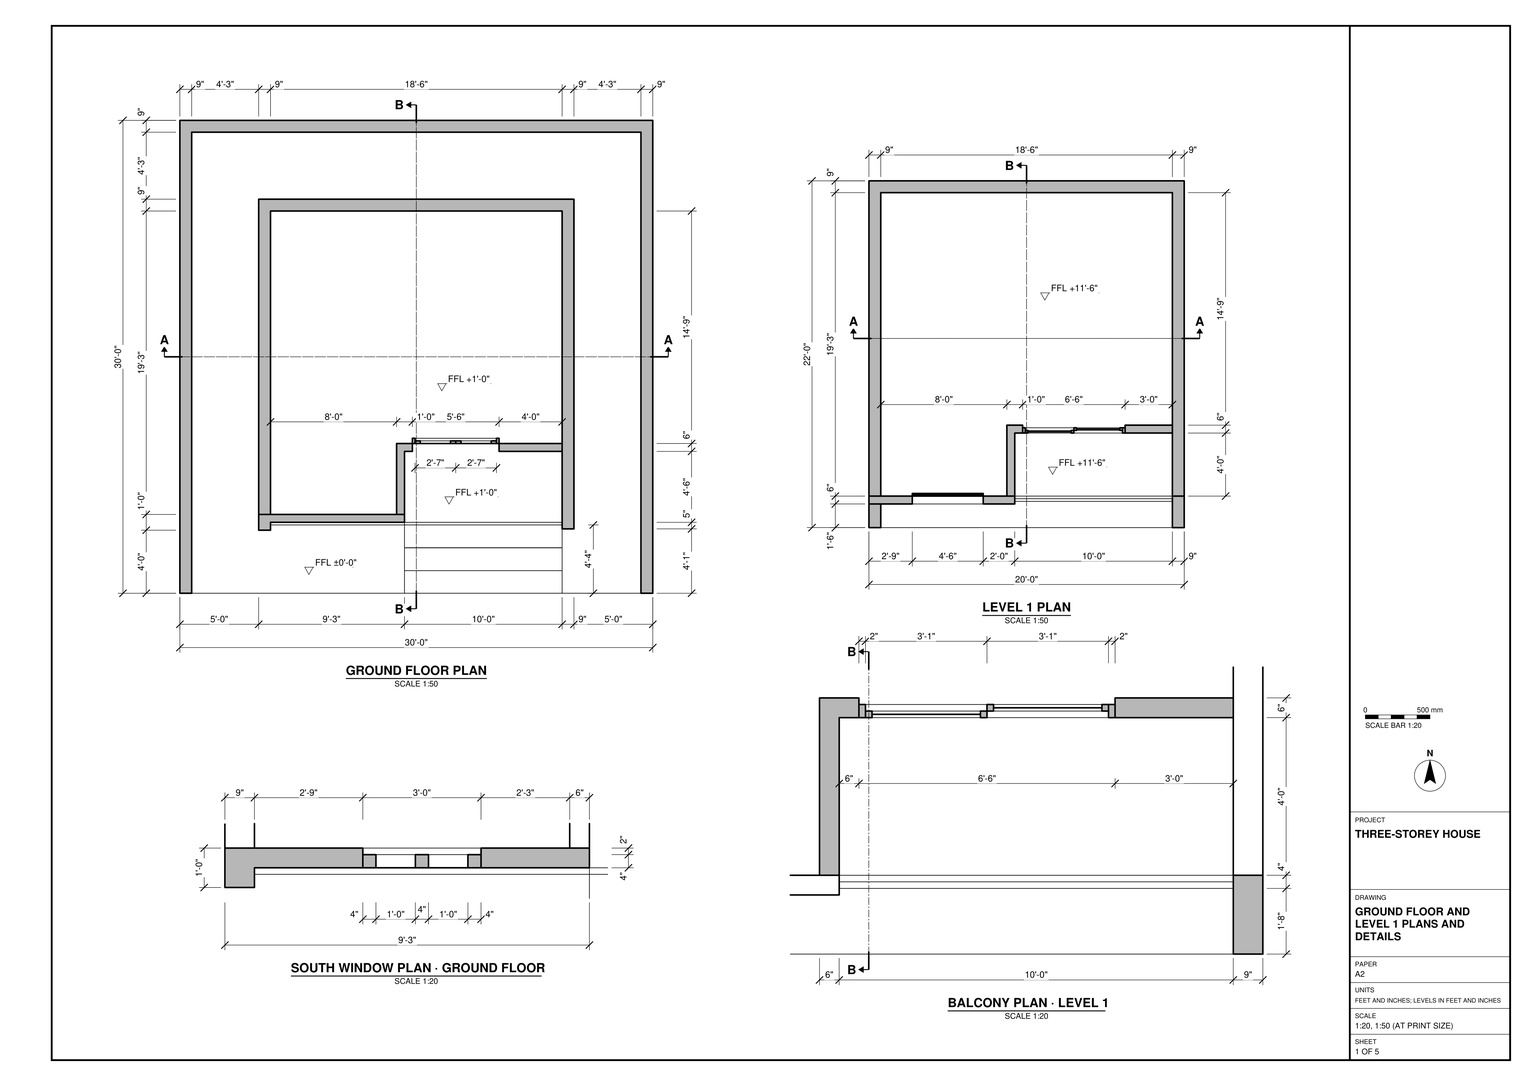
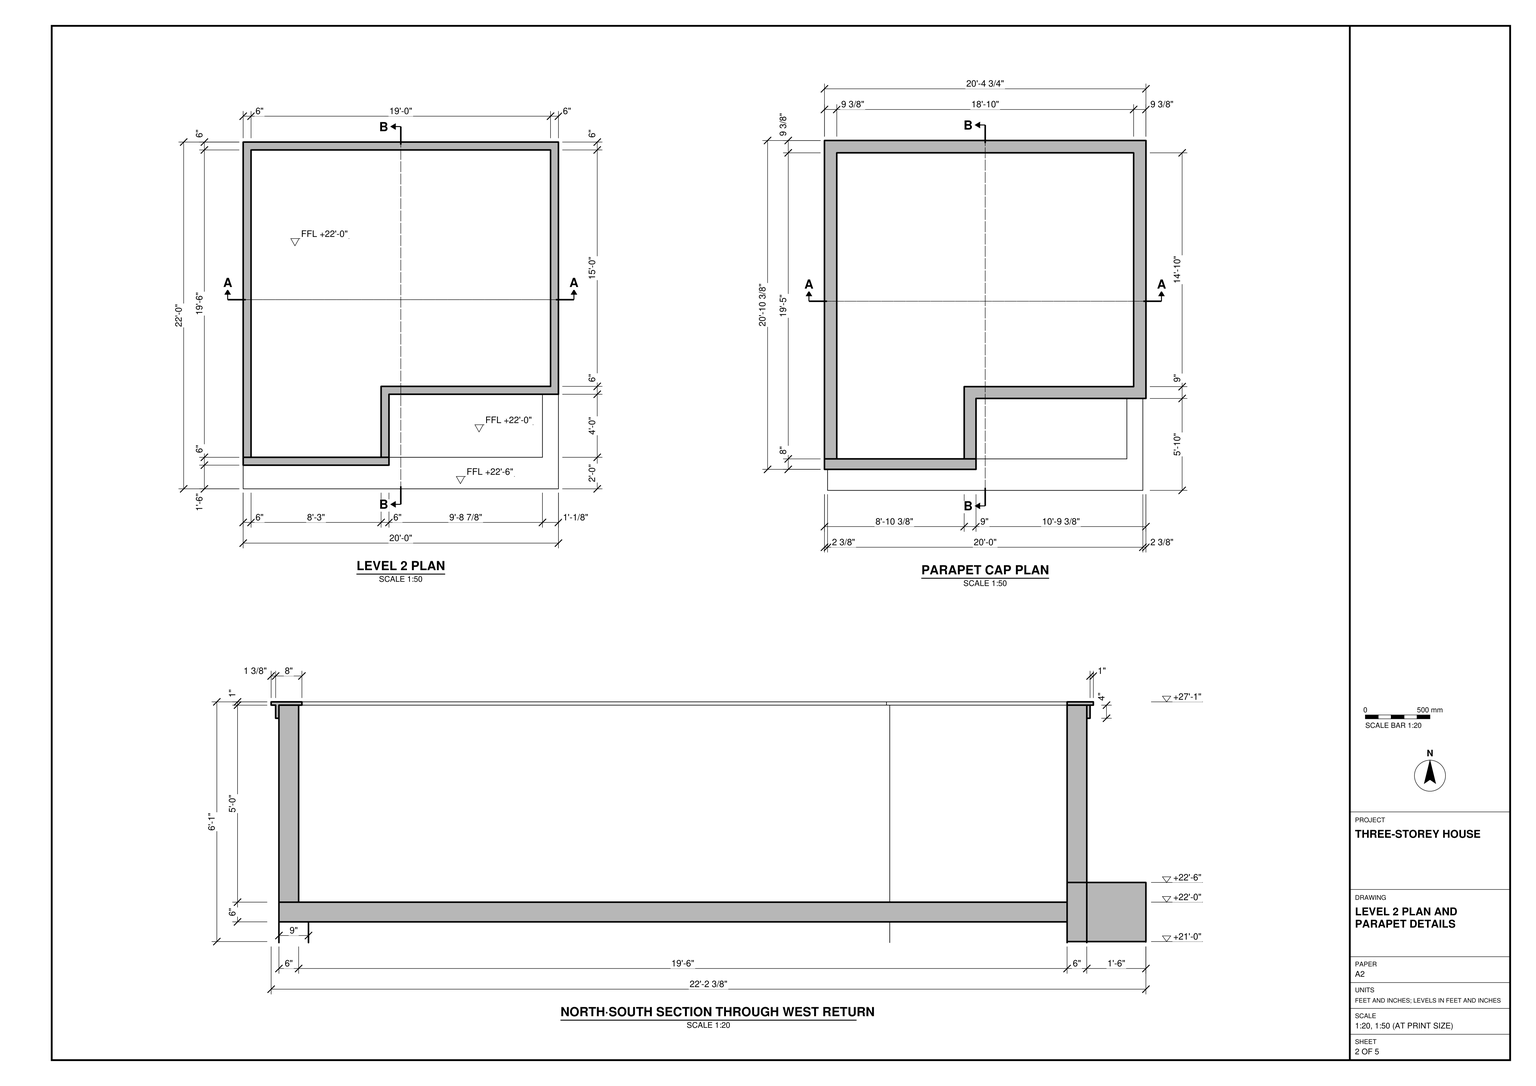
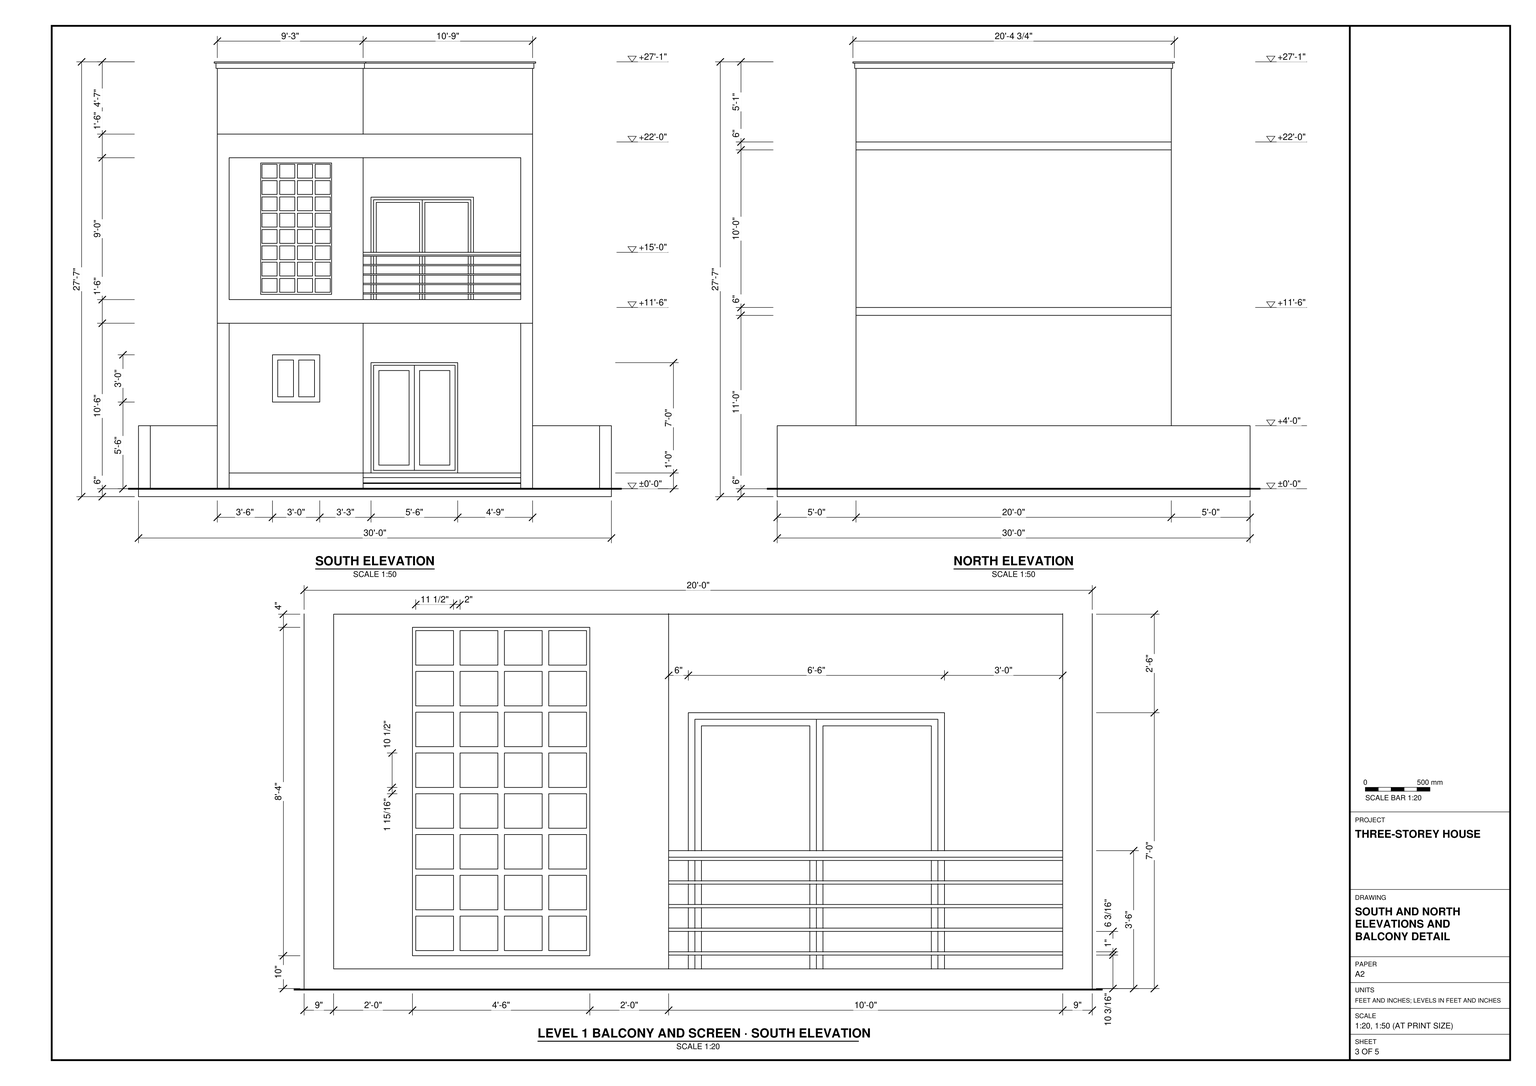
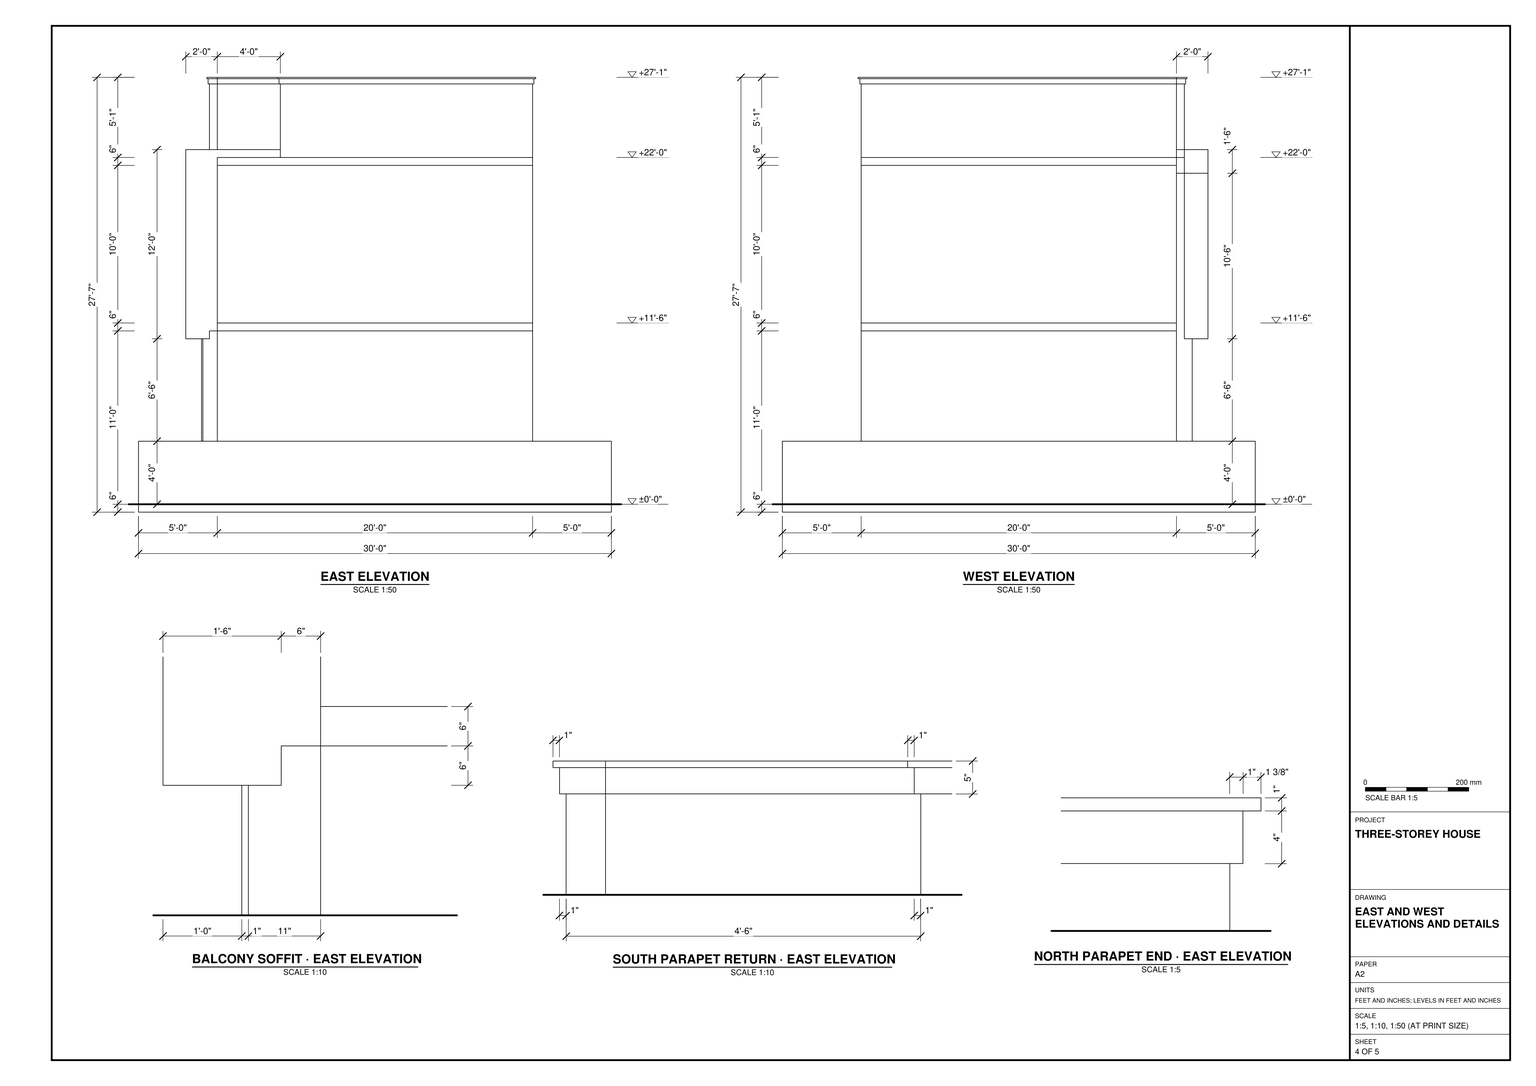
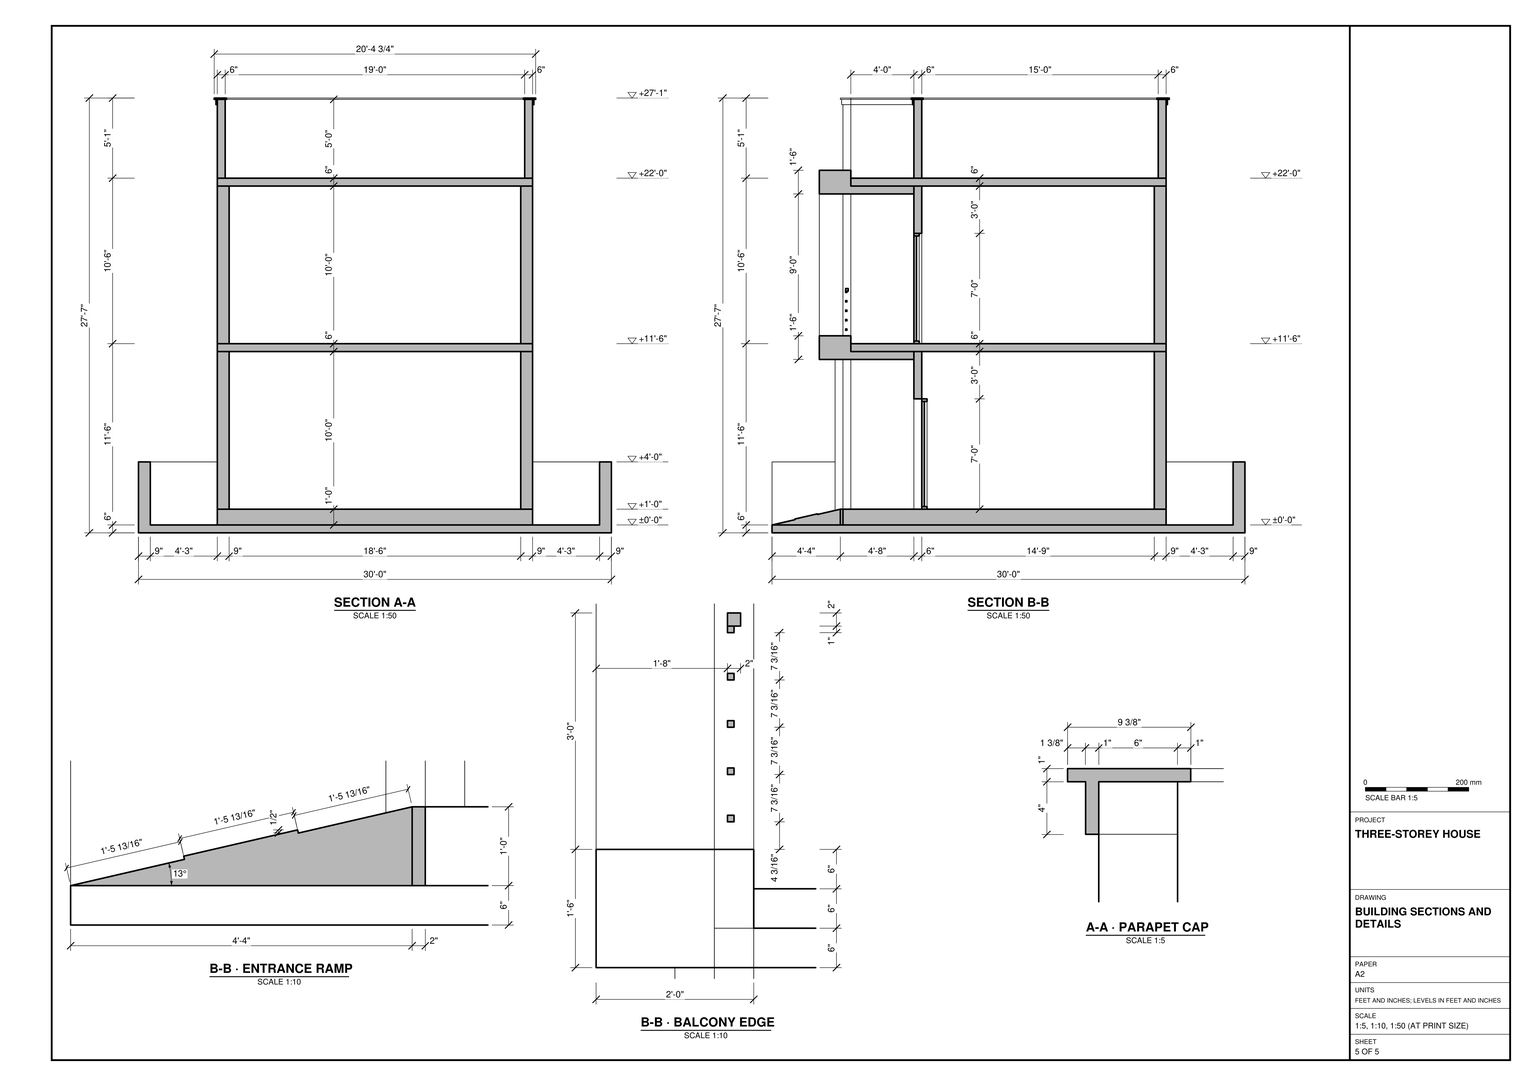
Build the house and its walled site in SketchUp from task_files/diagram_01.pdf. Work in feet and inches. The model is 30'-0" wide, 30'-0" deep and 27'-7" high, measured from the underside of the base slab to the top of the parapet cap. Use ±0'-0" as the ground datum, with Level 1 at +11'-6" and Level 2 at +22'-0". The finished ground floor is raised to +1'-0" above the approach.

Place the house between the low site walls, leaving the approach open to the south. Model the entrance steps, floor slabs and wall returns, following the wall thicknesses in plan. On the south face, place the small divided window to the left of the recessed entrance. Above it, build the tall grid screen beside the balcony, with the two-panel balcony doorway set back behind the horizontal railing. At roof level, follow the stepped parapet outline and carry the projecting cap around its returns.

Keep shell elements such as walls, slabs and roof, and each furniture or joinery piece shown, in separate groups or components. Use components for repeated parts. Any decor or loose items shown may be suitable library components. Save one SketchUp model as output_files/three_storey_house_with_a_recessed_south_balcony.skp.

# SketchUp Ruby script. Lengths in inches.
U = 1.inch
M = Sketchup.active_model
def pt(a) = Geom::Point3d.new(a.map { |v| v * U })
def face(e, loops, mat)
  f = e.add_face(loops[0].map { |a| pt(a) })
  loops[1..].each { |l| e.add_face(l.map { |a| pt(a) }).erase! }
  f.material = f.back_material = mat if mat
  f
end
# faces: each face lists its corners as indices into pts; further lists are holes
def faces(e, pts, list, mat = nil) = list.each { |f| face(e, (f[0].is_a?(Array) ? f : [f]).map { |l| l.map { |i| pts[i] } }, mat) }
# xy, xz, yz: faces in a plane at the given z, y or x. An outline is a flat list of corners, or four numbers for a rectangle; further outlines are holes
def ring(l) = l.size == 4 ? [[l[0], l[1]], [l[2], l[1]], [l[2], l[3]], [l[0], l[3]]] : l.each_slice(2).to_a
def flat(e, list, mat, &to3) = list.each { |f| face(e, (f[0].is_a?(Array) ? f : [f]).map { |l| ring(l).map { |u, v| to3.(u, v) } }, mat) }
def xy(e, z, list, mat = nil) = flat(e, list, mat) { |x, y| [x, y, z] }
def xz(e, y, list, mat = nil) = flat(e, list, mat) { |x, z| [x, y, z] }
def yz(e, x, list, mat = nil) = flat(e, list, mat) { |y, z| [x, y, z] }
def lines(e, pts, list) = list.each { |a, b| e.add_line(pt(pts[a]), pt(pts[b])) }
# prism: a flat outline (further loops are holes) pulled along v
def prism(e, loops, v, mat = nil)
  f = face(e, loops, mat); d = Geom::Vector3d.new(v.map { |x| x * U })
  f.pushpull(f.normal.samedirection?(d) ? d.length : -d.length)
end
def box(e, o, s, mat = nil) = prism(e, [[o, [o[0] + s[0], o[1], o[2]], [o[0] + s[0], o[1] + s[1], o[2]], [o[0], o[1] + s[1], o[2]]]], [0, 0, s[2]], mat)
def at(x, y, z, deg = 0) = Geom::Transformation.translation(pt([x, y, z])) * Geom::Transformation.rotation(ORIGIN, Z_AXIS, deg.degrees)
def axes(o, x, y, z) = Geom::Transformation.new([*x, 0, *y, 0, *z, 0, *pt(o).to_a, 1])
def part(name) = M.definitions.add(name)
# library, detail: a bought-in or finely detailed component or shape, given as its bounding box
def library(name, o, s) = part(name).tap { |d| box(d.entities, o, s) }
def detail(e, o, s) = box(e.add_group.entities, o, s)
def put(e, d, t, mat = nil) = e.add_instance(d, t).tap { |i| i.material = mat if mat }
def group(e, t, mat = nil) = e.add_group.tap { |g| g.transformation = t; g.material = mat if mat }.entities
root = M.entities
M.materials.add("[Black Lines 2]").color = [239, 239, 239]
M.materials.add("[Carpet Berber Pattern Gray]").color = [165, 165, 165]
M.materials.add("[Carpet Diamond Yellow]").color = [226, 217, 124]
M.materials.add("[Color M05]").color = [114, 114, 114]
M.materials.add("[Metal Seamed]").color = [118, 119, 115]
M.materials.add("[Roofing Slate Tan]1").color = [200, 175, 128]
M.materials.add("[Tile Travertine 2 inch]").color = [181, 178, 172]
M.materials.add("[Translucent Glass Blue]").color = [100, 149, 237]
M.materials["[Translucent Glass Blue]"].alpha = 0.5
M.materials.add("[Windmill]").color = [236, 236, 236]
M.materials.add("[Wood Floor]").color = [155, 105, 61]
c1 = library("Group\#10",[0,0,0],[54,2,100])
c2 = part("Group\#19")
xz(c2.entities,1,[[2,2,35,78]],"[Translucent Glass Blue]")
g1 = group(c2.entities,at(0,0,0))
prism(g1,[[[0,0,0],[37,0,0],[37,0,80],[0,0,80]],[[2,0,78],[35,0,78],[35,0,2],[2,0,2]]],[0,2,0])
prism(root,[[[171,0,6],[171,17.33,10],[171,17.22,10.49],[171,34.55,14.49],[171,34.67,14],[171,52,18],[171,52,6]]],[120,0,0],"[Tile Travertine 2 inch]")
p = [[171,54,18],[171,52,18]]
lines(root,p,[[0,1]])
g2 = group(root,at(0,0,0),"[Carpet Diamond Yellow]")
xy(g2,0,[[0,0,360,360]],"[Carpet Berber Pattern Gray]")
xy(g2,6,[[9,0,351,351]],"[Windmill]")
xy(g2,54,[[0,0,9,0,9,351,351,351,351,0,360,0,360,360,0,360]],"[Carpet Berber Pattern Gray]")
xz(g2,0,[[0,0,360,0,360,54,351,54,351,6,9,6,9,54,0,54]],"[Carpet Berber Pattern Gray]")
xz(g2,351,[[9,6,351,54]],"[Carpet Berber Pattern Gray]")
xz(g2,360,[[0,0,360,54]],"[Carpet Berber Pattern Gray]")
yz(g2,0,[[0,0,360,54]],"[Carpet Berber Pattern Gray]")
yz(g2,9,[[0,6,351,54]],"[Carpet Berber Pattern Gray]")
yz(g2,351,[[0,6,351,54]],"[Carpet Berber Pattern Gray]")
yz(g2,360,[[0,0,360,54]],"[Carpet Berber Pattern Gray]")
g3 = group(root,at(60,60,6),"[Color M05]")
xy(g3,0,[[0,-8,240,-6],[0,-6,240,240]])
xy(g3,12,[[0,-8,240,-6],[0,-6,240,240]])
xz(g3,-8,[[0,0,240,12]])
xz(g3,-6,[[0,0,240,12]])
xz(g3,240,[[0,0,240,12]])
yz(g3,0,[[-8,0,-6,12],[-6,0,240,12]])
yz(g3,240,[[-8,0,-6,12],[-6,0,240,12]])
g4 = group(root,at(60,60,18),"[Color M05]")
xy(g4,-12,[[231,-11,240,-8]])
xy(g4,0,[[231,-8,231,231,9,231,9,0,0,0,0,240,240,240,240,-8],[105,0,105,54,117,54,117,48,111,48,111,0],[183,48,231,54]])
xy(g4,84,[[117,48,183,54]])
xy(g4,114,[[231,-11,240,-6]])
xy(g4,120,[[231,-6,240,-6,240,240,0,240,0,0,9,0,9,231,231,231],[105,0,111,0,111,48,231,48,231,54,105,54]])
xz(g4,-11,[[231,-12,240,114]],"[Black Lines 2]")
xz(g4,-8,[[231,-12,240,0]])
xz(g4,-6,[[231,114,240,120]])
xz(g4,0,[[0,0,9,120],[105,0,111,120]])
xz(g4,48,[[111,0,117,0,117,84,183,84,183,0,231,0,231,120,111,120]])
xz(g4,54,[[105,0,105,120,231,120,231,0,183,0,183,84,117,84,117,0]])
xz(g4,231,[[9,0,231,120]])
xz(g4,240,[[0,0,240,120]])
yz(g4,0,[[0,0,240,120]])
yz(g4,9,[[0,0,231,120]])
yz(g4,105,[[0,0,54,120]])
yz(g4,111,[[0,0,48,120]])
yz(g4,117,[[48,0,54,84]])
yz(g4,183,[[48,0,54,84]])
yz(g4,231,[[48,0,54,120],[54,0,231,120],[-6,114,48,120]])
yz(g4,231,[[-11,-12,-11,114,48,114,48,0,-8,0,-8,-12]],"[Black Lines 2]")
yz(g4,240,[[0,0,240,120]])
yz(g4,240,[[-11,-12,-8,-12,-8,0,0,0,0,120,-6,120,-6,114,-11,114]],"[Black Lines 2]")
g5 = group(root,at(60,60,138),"[Color M05]")
box(g5,[0,0,0],[240,240,6])
g6 = group(root,at(60,60,264),"[Color M05]")
box(g6,[0,0,0],[240,240,6])
g7 = group(root,at(60,60,144),"[Color M05]")
xy(g7,0,[[0,0,0,240,240,240,240,0,231,0,231,231,9,231,9,0],[105,0,105,54,117,54,117,48,111,48,111,0],[195,48,231,54]])
xy(g7,84,[[117,48,195,54]])
xy(g7,120,[[0,0,9,0,9,231,231,231,231,0,240,0,240,240,0,240],[105,0,111,0,111,48,231,48,231,54,105,54]])
xz(g7,0,[[0,0,9,120],[105,0,111,120],[231,0,240,120]])
xz(g7,48,[[111,0,117,0,117,84,195,84,195,0,231,0,231,120,111,120]])
xz(g7,54,[[105,0,105,120,231,120,231,0,195,0,195,84,117,84,117,0]])
xz(g7,231,[[9,0,231,120]])
xz(g7,240,[[0,0,240,120]])
yz(g7,0,[[0,0,240,120]])
yz(g7,9,[[0,0,231,120]])
yz(g7,105,[[0,0,54,120]])
yz(g7,111,[[0,0,48,120]])
yz(g7,117,[[48,0,54,84]])
yz(g7,195,[[48,0,54,84]])
yz(g7,231,[[0,0,48,120],[48,0,54,120],[54,0,231,120]])
yz(g7,240,[[0,0,240,120]])
g8 = group(root,at(60,60,270),"[Black Lines 2]")
xy(g8,0,[[0,0,0,240,240,240,240,48,111,48,111,0,105,0,105,54,234,54,234,234,6,234,6,0]])
xy(g8,56,[[-1,0,-1,241,241,241,241,47,112,47,112,0,111,0,111,48,240,48,240,240,0,240,0,0]])
xy(g8,60,[[-2.375,0,-2.375,242.375,242.375,242.375,242.375,47,241,47,241,241,-1,241,-1,0],[0,0,0,240,240,240,240,48,111,48,111,0,105,0,105,54,234,54,234,234,6,234,6,0],[6,0,6,234,234,234,234,54,104,54,104,55,233,55,233,233,7,233,7,0],[104,0,105,54],[112,0,112,47,241,47,241,46,113,46,113,0],
  [241,46,242.375,47]])
xy(g8,61,[[-2.375,0,7,0,7,233,233,233,233,55,104,55,104,0,113,0,113,46,242.375,46,242.375,242.375,-2.375,242.375]])
xz(g8,0,[[0,0,6,60],[105,0,108,60],[108,0,111,60],[-1,56,0,56,0,60,7,60,7,61,-1,61],[111,56,112,61],
  [-2.375,60,-1,61],[104,60,108,61],[108,60,111,61],[112,60,113,61]])
xz(g8,46,[[113,60,242.375,61]])
xz(g8,47,[[112,56,241,60]])
xz(g8,48,[[111,56,240,60]])
xz(g8,48,[[111,0,240,56]],"[Color M05]")
xz(g8,54,[[105,0,234,60]],"[Color M05]")
xz(g8,55,[[104,60,233,61]])
xz(g8,233,[[7,60,233,61]])
xz(g8,234,[[6,0,234,60]],"[Color M05]")
xz(g8,240,[[0,56,240,60]])
xz(g8,240,[[0,0,240,56]],"[Color M05]")
xz(g8,241,[[-1,56,241,60]])
xz(g8,242.375,[[-2.375,60,242.375,61]])
yz(g8,-2.375,[[0,60,242.375,61]])
yz(g8,-1,[[0,56,241,60]])
yz(g8,0,[[0,56,240,60]])
yz(g8,0,[[0,0,240,56]],"[Color M05]")
yz(g8,6,[[0,0,234,60]],"[Color M05]")
yz(g8,7,[[0,60,233,61]])
yz(g8,104,[[0,60,55,61]])
yz(g8,105,[[0,0,54,60]],"[Color M05]")
yz(g8,111,[[0,56,48,60]])
yz(g8,111,[[0,0,48,56]],"[Color M05]")
yz(g8,112,[[0,56,47,60]])
yz(g8,113,[[0,60,46,61]])
yz(g8,233,[[55,60,233,61]])
yz(g8,234,[[54,0,234,60]],"[Color M05]")
yz(g8,240,[[48,56,240,60]])
yz(g8,240,[[48,0,240,56]],"[Color M05]")
yz(g8,241,[[47,56,241,60]])
yz(g8,242.375,[[46,60,242.375,61]])
p = [[105,0,0],[102,0,0],[-1,241,60],[-1,241,61]]
lines(g8,p,[[0,1],[2,3]])
g9 = group(root,at(60,36,132),"[Black Lines 2]")
xy(g9,0,[[0,0,0,18,111,18,111,72,231,72,231,18,240,18,240,0]])
xy(g9,6,[[231,18,240,24],[111,24,231,72]])
xy(g9,18,[[9,0,231,0,231,24,111,24,111,18,9,18]])
xy(g9,126,[[9,0,9,18,0,18,0,24,111,24,111,72,231,72,231,0]])
xy(g9,132,[[111,24,231,72]])
xy(g9,138,[[227.85,24,240,72]])
xy(g9,144,[[0,0,240,0,240,72,227.85,72,227.85,24,0,24]])
xz(g9,0,[[[0,0,240,144],[9,18,231,126]]])
xz(g9,18,[[0,0,0,126,9,126,9,18,111,18,111,0],[231,0,240,6]])
xz(g9,24,[[111,6,111,18,231,18,231,132,111,132,111,126,0,126,0,144,227.85,144,227.85,138,240,138,240,6]])
xz(g9,72,[[111,0,231,6],[111,126,231,132],[227.85,138,240,144]])
yz(g9,0,[[0,0,18,126],[0,126,24,144]])
yz(g9,9,[[0,18,18,126]])
yz(g9,111,[[18,0,72,6],[18,6,24,18],[24,126,72,132]])
yz(g9,227.85,[[24,138,72,144]])
yz(g9,231,[[18,0,72,6],[0,18,24,126],[24,126,72,132]])
yz(g9,240,[[0,0,18,0,18,6,24,6,24,138,72,138,72,144,0,144]])
put(root,c1,at(93,60,154),"[Metal Seamed]")
g10 = group(root,at(102,54,72),"[Metal Seamed]")
g11 = group(g10,at(0,0,0))
prism(g11,[[[36,4,0],[0,4,0],[0,4,36],[36,4,36]],[[32,4,32],[20,4,32],[20,4,4],[32,4,4]],[[16,4,4],[16,4,32],[4,4,32],[4,4,4]]],[0,-4,0])
p = [[20,4,32],[16,4,32]]
lines(g11,p,[[0,1]])
g12 = group(g10,at(20,0,4),"[Translucent Glass Blue]")
xz(g12,0,[[0,0,12,28]])
g13 = group(g10,at(4,0,4),"[Translucent Glass Blue]")
xz(g13,0,[[0,0,12,28]])
g14 = group(root,at(60,60,18),"[Black Lines 2]")
xy(g14,-12,[[0,-12,9,-8]])
xy(g14,0,[[0,-8,0,0,111,0,111,-6,9,-6,9,-8]])
xy(g14,54,[[42,-6,78,0]])
xy(g14,90,[[42,-6,78,0]])
xy(g14,114,[[0,-12,9,-6]])
xy(g14,136,[[33,-6,87,0]],"[Color M05]")
xy(g14,236,[[33,-6,87,0]],"[Color M05]")
xy(g14,308,[[-1,-7,-1,0,0,0,0,-6,111,-6,111,0,112,0,112,-7]])
xy(g14,312,[[-2.375,-8,113,-7],[-2.375,-7,-1,-6],[-1,-7,112,-6],[112,-7,113,-6],[-2.375,-6,-1,0],
  [-1,-6,0,0],[0,-6,111,0],[111,-6,112,0],[112,-6,113,0]])
xy(g14,313,[[-2.375,-8,113,0]])
xz(g14,-12,[[0,-12,9,114]])
xz(g14,-8,[[0,-12,9,0],[-2.375,312,113,313]])
xz(g14,-7,[[-1,308,112,312]])
xz(g14,-6,[[0,308,111,312]])
xz(g14,-6,[[[0,114,9,114,9,120,111,120,111,308,0,308],[33,136,87,236]]],"[Color M05]")
xz(g14,-6,[[[9,0,111,120],[42,54,78,90]]],"[Roofing Slate Tan]1")
xz(g14,0,[[[0,0,111,312],[33,136,87,236],[42,54,78,90]],[-1,308,0,312],[111,308,112,312],[-2.375,312,113,313]])
yz(g14,-2.375,[[-8,312,0,313]])
yz(g14,-1,[[-7,308,0,312]])
yz(g14,0,[[-12,-12,-12,114,-6,114,-6,252,0,252,0,0,-8,0,-8,-12],[-6,308,0,312]])
yz(g14,0,[[-6,252,0,308]],"[Color M05]")
yz(g14,9,[[-12,-12,-8,-12,-8,0,-6,0,-6,114,-12,114]])
yz(g14,33,[[-6,136,0,236]],"[Color M05]")
yz(g14,42,[[-6,54,0,90]])
yz(g14,78,[[-6,54,0,90]])
yz(g14,87,[[-6,136,0,236]],"[Color M05]")
yz(g14,111,[[-6,308,0,312]])
yz(g14,111,[[-6,120,0,308]],"[Color M05]")
yz(g14,111,[[-6,0,0,120]],"[Roofing Slate Tan]1")
yz(g14,112,[[-7,308,0,312]])
yz(g14,113,[[-8,312,0,313]])
g15 = group(root,at(177,114,18),"[Wood Floor]")
xz(g15,0,[[6,6,29,78],[37,6,60,78]],"[Translucent Glass Blue]")
g16 = group(g15,at(0,0,0),"[Wood Floor]")
xy(g16,0,[[0,0,66,4]])
xy(g16,2,[[2,0,33,2],[33,0,64,2],[2,2,64,4]])
xy(g16,6,[[6,0,29,2],[37,0,60,2]])
xy(g16,78,[[6,0,29,2],[37,0,60,2]])
xy(g16,82,[[2,0,33,2],[33,0,64,2],[2,2,64,4]])
xy(g16,84,[[0,0,66,4]])
xz(g16,0,[[[0,0,66,84],[2,2,64,82]],[[2,2,33,82],[6,6,29,78]],[[33,2,64,82],[37,6,60,78]]])
xz(g16,2,[[[2,2,33,82],[6,6,29,78]],[[33,2,64,82],[37,6,60,78]]])
xz(g16,4,[[[0,0,66,84],[2,2,64,82]]])
yz(g16,0,[[0,0,4,84]])
yz(g16,2,[[0,2,2,82],[2,2,4,82]])
yz(g16,6,[[0,6,2,78]])
yz(g16,29,[[0,6,2,78]])
yz(g16,33,[[0,2,2,82]])
yz(g16,37,[[0,6,2,78]])
yz(g16,60,[[0,6,2,78]])
yz(g16,64,[[0,2,2,82],[2,2,4,82]])
yz(g16,66,[[0,0,4,84]])
g17 = group(root,at(177,108,144))
put(g17,c2,at(39,2,2),"[Metal Seamed]")
g18 = group(g17,at(0,4,0),"[Metal Seamed]")
prism(g18,[[[78,0,0],[0,0,0],[0,0,84],[78,0,84]],[[2,0,2],[76,0,2],[76,0,82],[2,0,82]]],[0,-4,0])
put(g17,c2,at(2,0,2),"[Metal Seamed]")
g19 = group(root,at(171,56,154.2),"[Metal Seamed]")
g20 = group(g19,at(0,1,-6.2))
box(g20,[0,-1,6.2],[120,1,1])
box(g20,[0,-1,35],[120,1,1])
box(g20,[0,-1,13.4],[120,1,1])
box(g20,[0,-1,20.6],[120,1,1])
box(g20,[0,-1,27.8],[120,1,1])
g21 = group(g19,at(0,0,29.8))
box(g21,[0,0,0],[120,2,2])
